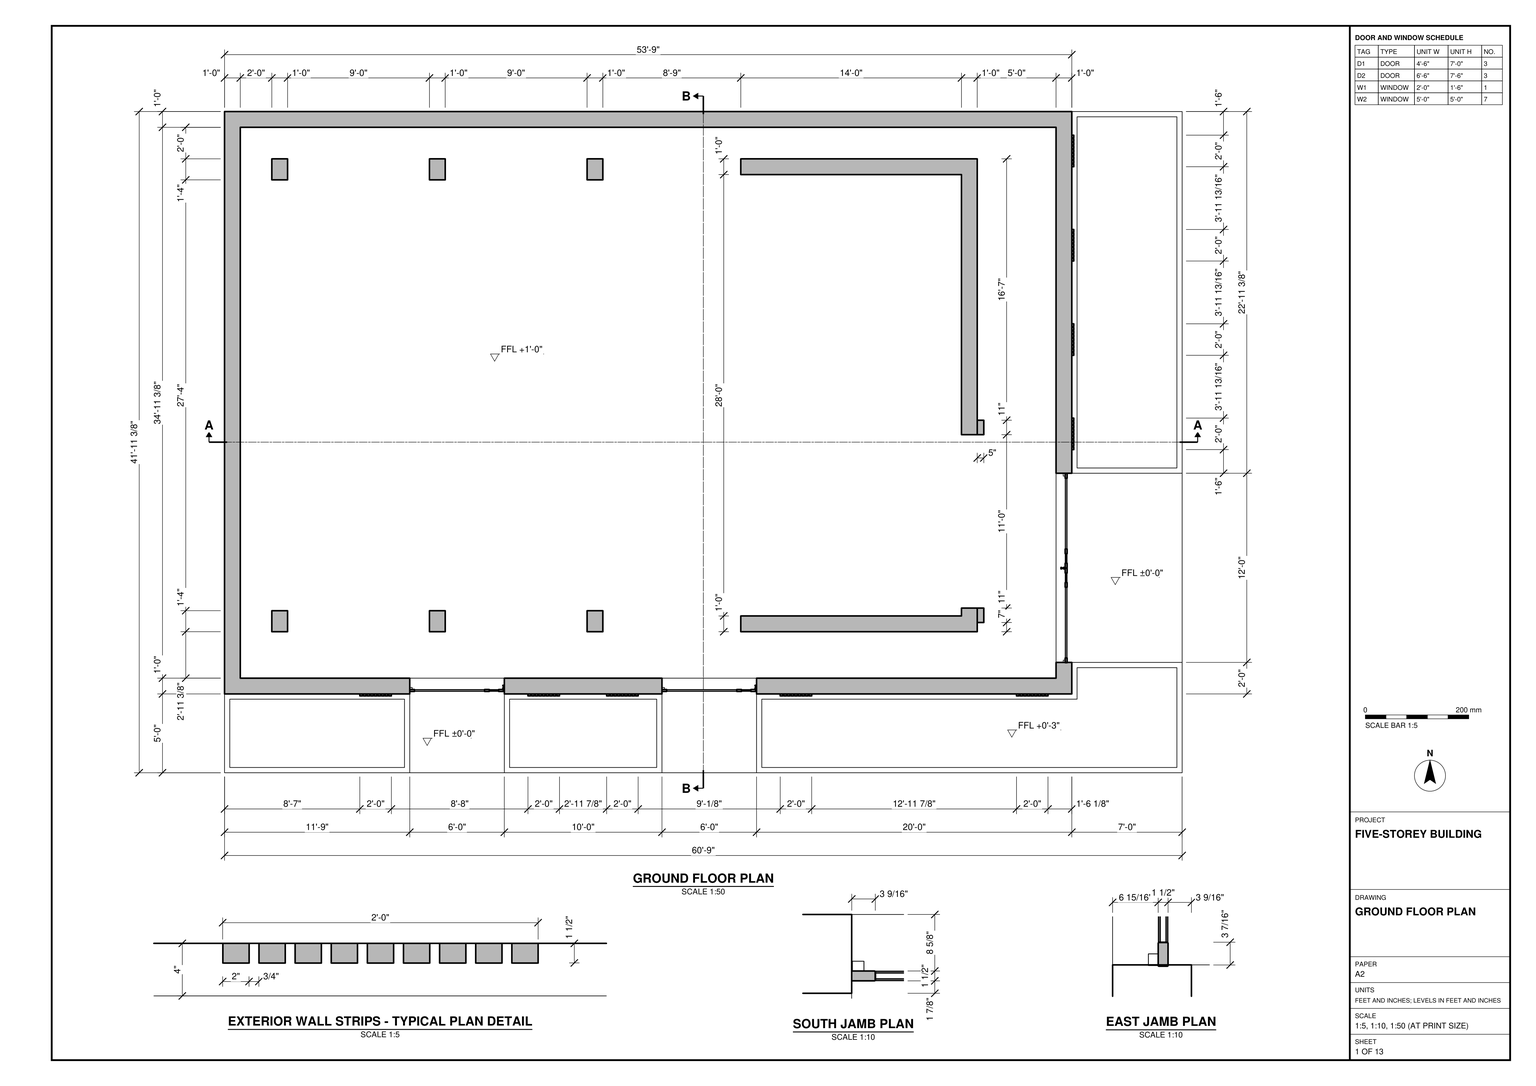
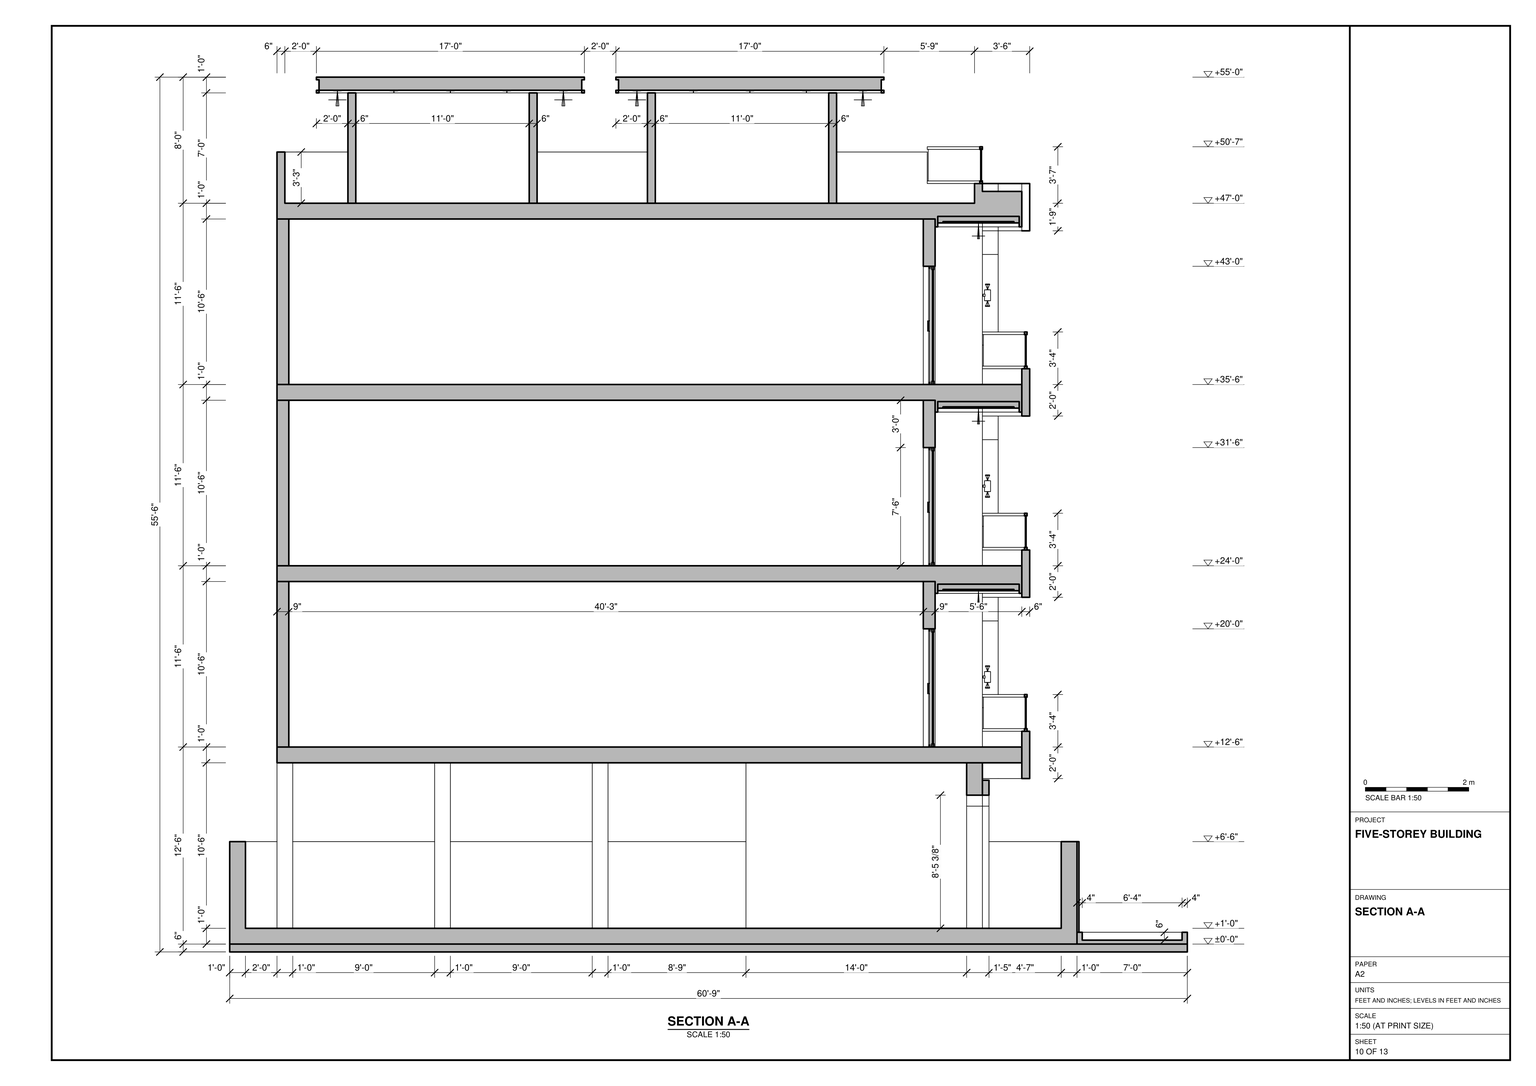
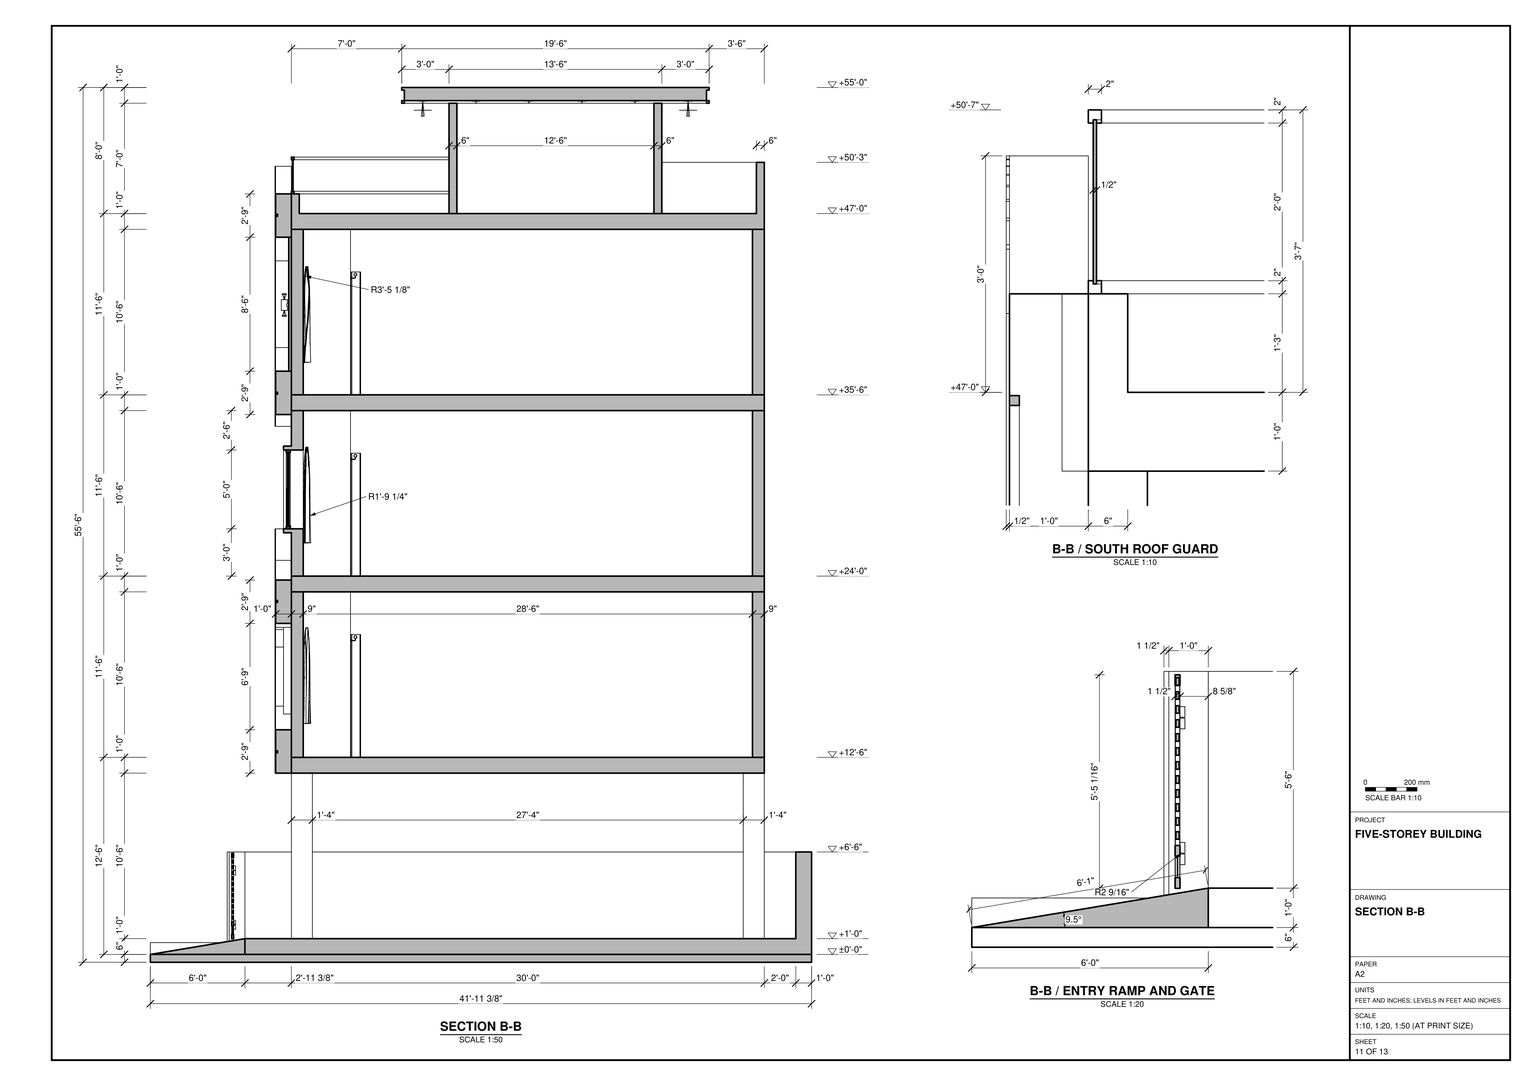
Build the building in SketchUp from task_files/diagram_01.pdf. Work in feet and inches. The complete model, including the base and rooftop canopies, measures 60'-9" east to west, 41'-11 3/8" north to south and 55'-6" from bottom to top. Use ±0'-0" as the ground datum and set the successive slab levels at +12'-6", +24'-0", +35'-6" and +47'-0". The last of these is the roof terrace, not the canopy top.

Start with the raised ground floor, low perimeter walls, entry ramps and gates. Keep the ground floor open around the two rows of freestanding columns, with the longer return wall and shorter wall in their plan positions to the east. Model the upper walls and slabs at the thicknesses drawn. Use the plans and opening schedule to place and size the doors and windows. Carry the east balconies beyond the enclosed floors and follow the sections for their slab edges and guards. On the roof, distinguish the solid parapets from the guarded edges and leave a gap between the two post-supported canopies. Include stairs, built-in joinery and main furniture only where shown on the sheets.

Keep walls, slabs, roof elements and each furniture or joinery piece in separate groups or components; use components for repeated parts. Decor and loose items may be any suitable library components. Save one SketchUp model as output_files/five_storey_building_with_balconies_and_roof_canopies.skp.

# SketchUp Ruby script. Lengths in inches.
U = 1.inch
M = Sketchup.active_model
def pt(a) = Geom::Point3d.new(a.map { |v| v * U })
def face(e, loops, mat)
  f = e.add_face(loops[0].map { |a| pt(a) })
  loops[1..].each { |l| e.add_face(l.map { |a| pt(a) }).erase! }
  f.material = f.back_material = mat if mat
  f
end
# faces: each face lists its corners as indices into pts; further lists are holes
def faces(e, pts, list, mat = nil) = list.each { |f| face(e, (f[0].is_a?(Array) ? f : [f]).map { |l| l.map { |i| pts[i] } }, mat) }
# xy, xz, yz: faces in a plane at the given z, y or x. An outline is a flat list of corners, or four numbers for a rectangle; further outlines are holes
def ring(l) = l.size == 4 ? [[l[0], l[1]], [l[2], l[1]], [l[2], l[3]], [l[0], l[3]]] : l.each_slice(2).to_a
def flat(e, list, mat, &to3) = list.each { |f| face(e, (f[0].is_a?(Array) ? f : [f]).map { |l| ring(l).map { |u, v| to3.(u, v) } }, mat) }
def xy(e, z, list, mat = nil) = flat(e, list, mat) { |x, y| [x, y, z] }
def xz(e, y, list, mat = nil) = flat(e, list, mat) { |x, z| [x, y, z] }
def yz(e, x, list, mat = nil) = flat(e, list, mat) { |y, z| [x, y, z] }
def lines(e, pts, list) = list.each { |a, b| e.add_line(pt(pts[a]), pt(pts[b])) }
# prism: a flat outline (further loops are holes) pulled along v
def prism(e, loops, v, mat = nil)
  f = face(e, loops, mat); d = Geom::Vector3d.new(v.map { |x| x * U })
  f.pushpull(f.normal.samedirection?(d) ? d.length : -d.length)
end
def box(e, o, s, mat = nil) = prism(e, [[o, [o[0] + s[0], o[1], o[2]], [o[0] + s[0], o[1] + s[1], o[2]], [o[0], o[1] + s[1], o[2]]]], [0, 0, s[2]], mat)
def at(x, y, z, deg = 0) = Geom::Transformation.translation(pt([x, y, z])) * Geom::Transformation.rotation(ORIGIN, Z_AXIS, deg.degrees)
def axes(o, x, y, z) = Geom::Transformation.new([*x, 0, *y, 0, *z, 0, *pt(o).to_a, 1])
def part(name) = M.definitions.add(name)
# library, detail: a bought-in or finely detailed component or shape, given as its bounding box
def library(name, o, s) = part(name).tap { |d| box(d.entities, o, s) }
def detail(e, o, s) = box(e.add_group.entities, o, s)
def put(e, d, t, mat = nil) = e.add_instance(d, t).tap { |i| i.material = mat if mat }
def group(e, t, mat = nil) = e.add_group.tap { |g| g.transformation = t; g.material = mat if mat }.entities
root = M.entities
M.materials.add("1111 AP 9939 Brown seed-N").color = [120, 84, 73]
M.materials.add("1432 AP 8245 TAR ROAD").color = [71, 72, 75]
M.materials.add("Generic").color = [172, 166, 153]
M.materials.add("W142X827B75_NILAYA IMAGINE 31756 ROLL B75").color = [192, 192, 189]
M.materials.add("[Brick Tumbled]").color = [135, 132, 132]
M.materials.add("[Granite Dark Gray]").color = [69, 68, 68]
M.materials.add("[Tile Travertine 2 inch]").color = [181, 178, 172]
M.materials.add("[Wood Cherry Original]").color = [152, 86, 42]
M.materials.add("[Wood Veneer 01]").color = [120, 70, 37]
c1 = library("BathRoom Window",[2.44,2.32,-1.4375],[28.18,2.86,36])
c2 = library("WALL LIGHT 69",[4.19,4.05,-8.78],[4.61,5.7,17.13])
c3 = library("2",[-24,-36,-9.91],[204,234,21.91])
c4 = library("Double slatted gate",[7.03,-128.55,-3.91],[5.33,99.02,60.06])
c5 = part("5")
box(c5.entities,[0,0,0],[12,16,126])
c6 = library("Group\#10",[-12,-12.5,-12],[99,12.5,186])
c7 = library("Double-hung window 69 in. x 58 in. triple row with mullions",[0,0,-3.59],[62,58,4.59])
c8 = library("Glass Door",[0,0,0],[72,3.54,96])
c9 = library("RIDEAUX \#16",[0,0,0],[103.86,7.74,93.57])
c10 = library("Curtain",[0,0,0],[121.12,7.86,100.24])
c11 = library("SLIDING+GLASS+DOOR",[0,-0.75,0],[72,5.75,80])
c12 = library("Group\#19",[0,0,0],[0.5,51,105])
c13 = library("Group\#46",[0,-2,0],[168,2,149.16])
c14 = library("Group\#20",[0,0,0],[0.5,51,102])
c15 = library("Group\#21",[0,0,0],[0.5,51,102])
c16 = library("Group\#58",[0,0,-17.09],[62,80,17.09])
c17 = library("Group\#32",[0,0,-17.09],[62,80,17.09])
c18 = library("Group\#56",[0,0,-17.09],[62,80,17.09])
c19 = library("Group\#9",[-9,-13,-20.09],[567,364,75.09])
c20 = library("Group\#3",[-12,-12.5,-24],[99,12.5,198])
c21 = library("Group\#17",[0,0,-12],[36,360,453])
c22 = library("Group\#13",[0,-12,0],[330,12,441])
c23 = library("Group\#18",[0,0,-453],[48,48,453])
c24 = library("Group\#45",[0,-2,0],[63,2,36])
c25 = library("Group\#43",[0,-2,0],[63,2,36])
c26 = library("Group\#47",[0,0,0],[34,92,28])
c27 = library("Group\#64",[0,-1.5,0],[24,1.5,78])
c28 = part("Group\#66")
prism(c28.entities,[[[0,-72,0],[0,0,12],[0,0,0]]],[72,0,0])
c29 = library("Group\#62",[0,0,0],[185,360,126])
c30 = library("Group\#1077",[59.37,-1.74,0],[60.38,4.74,59.75])
g1 = group(root,at(21,107.37,1.59))
g2 = group(g1,at(0,0,166.2))
box(g2,[-21,-107.37,-156],[729,503.37,6],"[Brick Tumbled]")
put(g2,c1,axes([456.92,-1.16,234.72],[0.85182,0,0],[0,0.5,0],[0,0,0.5]))
put(g2,c2,at(464.24,-13.25,184.26))
put(g2,c2,at(464.24,-13.25,328.62))
put(g2,c2,at(298.46,-11.75,344.61))
put(g2,c2,at(262.52,-9.75,203.46))
put(g2,c2,at(360.51,-9.75,62.87))
put(g2,c2,at(127.76,-9.75,62.87))
put(g2,c2,at(127.76,-9.75,193.87))
put(g2,c2,at(562.25,55.625,344.18,90))
put(g2,c2,at(562.25,55.625,198.87,90))
put(g2,c2,at(562.25,55.625,53.55,90))
put(g2,c2,at(562.25,268.01,344.18,90))
put(g2,c2,at(562.25,268.01,198.87,90))
put(g2,c2,at(562.25,268.01,53.55,90))
put(g2,c3,at(69,120,498))
put(g2,c3,at(297,120,498))
put(g2,c4,axes([628.05,163.36,-133.82],[-1,0,0],[0,1.45416,0],[0,0,1.06965]))
put(g2,c5,at(15,0,-138),"W142X827B75_NILAYA IMAGINE 31756 ROLL B75")
put(g2,c5,at(15,344,-138),"W142X827B75_NILAYA IMAGINE 31756 ROLL B75")
put(g2,c5,at(135,0,-138),"W142X827B75_NILAYA IMAGINE 31756 ROLL B75")
put(g2,c5,at(135,344,-138),"W142X827B75_NILAYA IMAGINE 31756 ROLL B75")
put(g2,c5,at(255,0,-138),"W142X827B75_NILAYA IMAGINE 31756 ROLL B75")
put(g2,c5,at(255,344,-138),"W142X827B75_NILAYA IMAGINE 31756 ROLL B75")
put(g2,c6,at(24,0,0),"[Wood Veneer 01]")
g3 = group(g2,at(15,-6,279))
xy(g3,-3,[[0,6,9,366],[93,6,537,15],[93,15,102,51],[528,15,528,135,492,135,492,147,501,147,501,144,537,144,537,15],[9,42,24,51],
  [78,42,93,51],[492,225,492,237,528,237,528,357,537,357,537,228,501,228,501,225],[9,357,537,366]])
xy(g3,30,[[138,0,204,6],[330,0,396,6]],"1111 AP 9939 Brown seed-N")
xy(g3,33,[[141,0,201,15],[333,0,393,15]],"1111 AP 9939 Brown seed-N")
xy(g3,81,[[24,42,78,51]])
xy(g3,87,[[492,147,501,225]])
xy(g3,93,[[333,0,393,15]])
xy(g3,93,[[141,0,201,15]],"1111 AP 9939 Brown seed-N")
xy(g3,96,[[138,0,204,6],[330,0,396,6]],"1111 AP 9939 Brown seed-N")
xy(g3,123,[[[0,6,9,6,9,42,93,42,93,6,537,6,537,144,501,144,501,228,537,228,537,366,0,366],[102,15,102,51,9,51,9,357,528,357,528,237,492,237,492,135,528,135,528,15]]])
xz(g3,0,[[[138,30,204,96],[141,33,201,93]],[[330,30,396,96],[333,33,393,93]]],"1111 AP 9939 Brown seed-N")
xz(g3,6,[[0,-3,9,123],[[93,-3,537,123],[330,30,396,96],[138,30,204,96]]])
xz(g3,15,[[[102,-3,528,123],[141,33,201,93],[333,33,393,93]]])
xz(g3,42,[[9,-3,24,-3,24,81,78,81,78,-3,93,-3,93,123,9,123]])
xz(g3,51,[[9,-3,9,123,102,123,102,-3,78,-3,78,81,24,81,24,-3]])
xz(g3,135,[[492,-3,528,123]])
xz(g3,144,[[501,-3,537,123]])
xz(g3,147,[[492,-3,501,87]])
xz(g3,225,[[492,-3,501,87]])
xz(g3,228,[[501,-3,537,123]])
xz(g3,237,[[492,-3,528,123]])
xz(g3,357,[[9,-3,528,123]])
xz(g3,366,[[0,-3,537,123]])
yz(g3,0,[[6,-3,366,123]])
yz(g3,9,[[6,-3,42,123],[51,-3,357,123]])
yz(g3,24,[[42,-3,51,81]])
yz(g3,78,[[42,-3,51,81]])
yz(g3,93,[[6,-3,42,123]])
yz(g3,102,[[15,-3,51,123]])
yz(g3,138,[[0,30,6,96]],"1111 AP 9939 Brown seed-N")
yz(g3,141,[[0,33,15,93]],"1111 AP 9939 Brown seed-N")
yz(g3,201,[[0,33,15,93]],"1111 AP 9939 Brown seed-N")
yz(g3,204,[[0,30,6,96]])
yz(g3,330,[[0,30,6,96]],"1111 AP 9939 Brown seed-N")
yz(g3,333,[[0,33,15,93]],"1111 AP 9939 Brown seed-N")
yz(g3,393,[[0,33,15,93]],"1111 AP 9939 Brown seed-N")
yz(g3,396,[[0,30,6,96]],"1111 AP 9939 Brown seed-N")
yz(g3,492,[[135,-3,135,123,237,123,237,-3,225,-3,225,87,147,87,147,-3]])
yz(g3,501,[[144,-3,147,-3,147,87,225,87,225,-3,228,-3,228,123,144,123]])
yz(g3,528,[[15,-3,135,123],[237,-3,357,123]])
yz(g3,537,[[59.76,9,93,9,93,114,59.76,114,59.53,113.99,59.29,113.99,59.06,113.98,58.82,113.96,58.59,113.94,58.35,113.92,58.12,113.9,57.88,113.875,57.65,113.85,57.42,113.8125,57.18,113.78,56.72,113.7,56.49,113.65,56.26,113.61,56.03,113.56,55.8,113.5,55.57,113.45,55.34,113.39,55.11,113.32,54.89,113.26,54.66,113.19,54.4375,113.12,54.21,113.04,53.99,112.97,53.77,112.89,53.55,112.8,53.33,112.72,52.89,112.54,52.68,112.44,52.46,112.35,52.25,112.25,52.04,112.14,51.83,112.04,51.41,111.82,51.2,111.7,51,111.59,50.6,111.35,50.39,111.22,50.2,111.1,50,110.97,49.8,110.83,49.61,110.7,49.42,110.5625,49.23,110.42,49.04,110.28,48.86,110.14,48.67,109.99,48.49,109.84,48.31,109.6875,48.13,109.53,47.96,109.375,47.78,109.22,47.61,109.06,47.44,108.89,47.27,108.73,47.11,108.56,46.94,108.39,46.78,108.22,46.625,108.04,46.47,107.87,46.3125,107.69,46.16,107.51,46.01,107.33,45.86,107.14,45.72,106.96,45.58,106.77,45.4375,106.58,45.3,106.39,45.17,106.2,45.03,106,44.9,105.8,44.78,105.61,44.65,105.4,44.41,105,44.3,104.8,44.18,104.59,43.96,104.17,43.86,103.96,43.75,103.75,43.65,103.54,43.56,103.32,43.46,103.11,43.28,102.67,43.2,102.45,43.11,102.23,43.03,102.01,42.96,101.79,42.88,101.5625,42.81,101.34,42.74,101.11,42.68,100.89,42.61,100.66,42.55,100.43,42.5,100.2,42.44,99.97,42.39,99.74,42.35,99.51,42.3,99.28,42.22,98.82,42.1875,98.58,42.15,98.35,42.125,98.12,42.1,97.88,42.08,97.65,42.06,97.41,42.04,97.18,42.02,96.94,42.01,96.71,42.01,96.47,42,96.24,42,26.76,42.01,26.53,42.01,26.29,42.02,26.06,42.04,25.82,42.06,25.59,42.08,25.35,42.1,25.12,42.125,24.88,42.15,24.65,42.1875,24.42,42.22,24.18,42.3,23.72,42.35,23.49,42.39,23.26,42.44,23.03,42.5,22.8,42.55,22.57,42.61,22.34,42.68,22.11,42.74,21.89,42.81,21.66,42.88,21.4375,42.96,21.21,43.03,20.99,43.11,20.77,43.2,20.55,43.28,20.33,43.46,19.89,43.56,19.68,43.65,19.46,43.75,19.25,43.86,19.04,43.96,18.83,44.18,18.41,44.3,18.2,44.41,18,44.65,17.6,44.78,17.39,44.9,17.2,45.03,17,45.17,16.8,45.3,16.61,45.4375,16.42,45.58,16.23,45.72,16.04,45.86,15.86,46.01,15.67,46.16,15.49,46.3125,15.31,46.47,15.13,46.625,14.96,46.78,14.78,46.94,14.61,47.11,14.44,47.27,14.27,47.44,14.11,47.61,13.94,47.78,13.78,47.96,13.625,48.13,13.47,48.31,13.3125,48.49,13.16,48.67,13.01,48.86,12.86,49.04,12.72,49.23,12.58,49.42,12.4375,49.61,12.3,49.8,12.17,50,12.03,50.2,11.9,50.39,11.78,50.6,11.65,51,11.41,51.2,11.3,51.41,11.18,51.83,10.96,52.04,10.86,52.25,10.75,52.46,10.65,52.68,10.56,52.89,10.46,53.33,10.28,53.55,10.2,53.77,10.11,53.99,10.03,54.21,9.96,54.4375,9.88,54.66,9.81,54.89,9.74,55.11,9.68,55.34,9.61,55.57,9.55,55.8,9.5,56.03,9.44,56.26,9.39,56.49,9.35,56.72,9.3,57.18,9.22,57.42,9.1875,57.65,9.15,57.88,9.125,58.12,9.1,58.35,9.08,58.59,9.06,58.82,9.04,59.06,9.02,59.29,9.01,59.53,9.01]])
yz(g3,537,[[[6,-3,144,123],[59.76,9,59.53,9.01,59.29,9.01,59.06,9.02,58.82,9.04,58.59,9.06,58.35,9.08,58.12,9.1,57.88,9.125,57.65,9.15,57.42,9.1875,57.18,9.22,56.72,9.3,56.49,9.35,56.26,9.39,56.03,9.44,55.8,9.5,55.57,9.55,55.34,9.61,55.11,9.68,54.89,9.74,54.66,9.81,54.4375,9.88,54.21,9.96,53.99,10.03,53.77,10.11,53.55,10.2,53.33,10.28,52.89,10.46,52.68,10.56,52.46,10.65,52.25,10.75,52.04,10.86,51.83,10.96,51.41,11.18,51.2,11.3,51,11.41,50.6,11.65,50.39,11.78,50.2,11.9,50,12.03,49.8,12.17,49.61,12.3,49.42,12.4375,49.23,12.58,49.04,12.72,48.86,12.86,48.67,13.01,48.49,13.16,48.31,13.3125,48.13,13.47,47.96,13.625,47.78,13.78,47.61,13.94,47.44,14.11,47.27,14.27,47.11,14.44,46.94,14.61,46.78,14.78,46.625,14.96,46.47,15.13,46.3125,15.31,46.16,15.49,46.01,15.67,45.86,15.86,45.72,16.04,45.58,16.23,45.4375,16.42,45.3,16.61,45.17,16.8,45.03,17,44.9,17.2,44.78,17.39,44.65,17.6,44.41,18,44.3,18.2,44.18,18.41,43.96,18.83,43.86,19.04,43.75,19.25,43.65,19.46,43.56,19.68,43.46,19.89,43.28,20.33,43.2,20.55,43.11,20.77,43.03,20.99,42.96,21.21,42.88,21.4375,42.81,21.66,42.74,21.89,42.68,22.11,42.61,22.34,42.55,22.57,42.5,22.8,42.44,23.03,42.39,23.26,42.35,23.49,42.3,23.72,42.22,24.18,42.1875,24.42,42.15,24.65,42.125,24.88,42.1,25.12,42.08,25.35,42.06,25.59,42.04,25.82,42.02,26.06,42.01,26.29,42.01,26.53,42,26.76,42,96.24,42.01,96.47,42.01,96.71,42.02,96.94,42.04,97.18,42.06,97.41,42.08,97.65,42.1,97.88,42.125,98.12,42.15,98.35,42.1875,98.58,42.22,98.82,42.3,99.28,42.35,99.51,42.39,99.74,42.44,99.97,42.5,100.2,42.55,100.43,42.61,100.66,42.68,100.89,42.74,101.11,42.81,101.34,42.88,101.5625,42.96,101.79,43.03,102.01,43.11,102.23,43.2,102.45,43.28,102.67,43.46,103.11,43.56,103.32,43.65,103.54,43.75,103.75,43.86,103.96,43.96,104.17,44.18,104.59,44.3,104.8,44.41,105,44.65,105.4,44.78,105.61,44.9,105.8,45.03,106,45.17,106.2,45.3,106.39,45.4375,106.58,45.58,106.77,45.72,106.96,45.86,107.14,46.01,107.33,46.16,107.51,46.3125,107.69,46.47,107.87,46.625,108.04,46.78,108.22,46.94,108.39,47.11,108.56,47.27,108.73,47.44,108.89,47.61,109.06,47.78,109.22,47.96,109.375,48.13,109.53,48.31,109.6875,48.49,109.84,48.67,109.99,48.86,110.14,49.04,110.28,49.23,110.42,49.42,110.5625,49.61,110.7,49.8,110.83,50,110.97,50.2,111.1,50.39,111.22,50.6,111.35,51,111.59,51.2,111.7,51.41,111.82,51.83,112.04,52.04,112.14,52.25,112.25,52.46,112.35,52.68,112.44,52.89,112.54,53.33,112.72,53.55,112.8,53.77,112.89,53.99,112.97,54.21,113.04,54.4375,113.12,54.66,113.19,54.89,113.26,55.11,113.32,55.34,113.39,55.57,113.45,55.8,113.5,56.03,113.56,56.26,113.61,56.49,113.65,56.72,113.7,57.18,113.78,57.42,113.8125,57.65,113.85,57.88,113.875,58.12,113.9,58.35,113.92,58.59,113.94,58.82,113.96,59.06,113.98,59.29,113.99,59.53,113.99,59.76,114,93,114,93,9]],[228,-3,366,123]],"Generic")
put(g3,c7,axes([201,4.5,33],[-0.96774,0,0],[0,0,1.03448],[0,0.696,0]),"[Granite Dark Gray]")
put(g3,c7,axes([393,4.5,33],[-0.96774,0,0],[0,0,1.03448],[0,0.696,0]),"[Granite Dark Gray]")
put(g3,c8,axes([24,42,-3],[0.75,0,0],[0,0.74,0],[0,0,0.875]))
put(g3,c9,axes([9,51,-3],[0.79912,0,0],[0,1,0],[0,0,1]))
put(g3,c10,axes([126.82,15,21.67],[0.73,0,0],[0,0.73,0],[0,0,0.73]))
put(g3,c10,axes([314.2,15,21.67],[0.73,0,0],[0,0.73,0],[0,0,0.73]))
put(g3,c11,axes([496,225,-3],[0,-1.08333,0],[1,0,0],[0,0,1.125]))
put(g3,c12,at(537,42,9),"[Wood Veneer 01]")
put(g3,c13,at(240,6,-32.16),"Generic")
g4 = group(g2,at(15,-6,141))
xy(g4,-3,[[0,6,0,366,528,366,528,357,9,357,9,51,24,51,24,42,9,42,9,6],[93,6,93,42,78,42,78,51,102,51,102,15,528,15,528,135,492,135,492,147,501,147,501,144,537,144,537,6],[492,225,492,237,528,237,528,366,537,366,537,228,501,228,501,225]])
xy(g4,30,[[138,0,204,6],[306,0,372,6]],"1111 AP 9939 Brown seed-N")
xy(g4,33,[[141,0,201,15],[309,0,369,15]],"1111 AP 9939 Brown seed-N")
xy(g4,81,[[24,42,78,51]])
xy(g4,87,[[492,147,501,225]])
xy(g4,93,[[444,6,468,15]])
xy(g4,93,[[141,0,201,15],[309,0,369,15]],"1111 AP 9939 Brown seed-N")
xy(g4,96,[[138,0,204,6],[306,0,372,6]],"1111 AP 9939 Brown seed-N")
xy(g4,111,[[444,6,468,15]])
xy(g4,123,[[[0,6,9,6,9,42,93,42,93,6,537,6,537,144,501,144,501,228,537,228,537,366,0,366],[102,15,102,51,9,51,9,357,528,357,528,237,492,237,492,135,528,135,528,15]]])
xz(g4,0,[[[138,30,204,96],[141,33,201,93]],[[306,30,372,96],[309,33,369,93]]],"1111 AP 9939 Brown seed-N")
xz(g4,6,[[0,-3,9,123],[[93,-3,537,123],[138,30,204,96],[306,30,372,96],[444,93,468,111]]])
xz(g4,15,[[[102,-3,528,123],[309,33,369,93],[141,33,201,93],[444,93,468,111]]])
xz(g4,42,[[9,-3,24,-3,24,81,78,81,78,-3,93,-3,93,123,9,123]])
xz(g4,51,[[9,-3,9,123,102,123,102,-3,78,-3,78,81,24,81,24,-3]])
xz(g4,135,[[492,-3,528,123]])
xz(g4,144,[[501,-3,537,123]])
xz(g4,147,[[492,-3,501,87]])
xz(g4,225,[[492,-3,501,87]])
xz(g4,228,[[501,-3,537,123]])
xz(g4,237,[[492,-3,528,123]])
xz(g4,357,[[9,-3,528,123]])
xz(g4,366,[[0,-3,537,123]])
yz(g4,0,[[6,-3,366,123]])
yz(g4,9,[[6,-3,42,123],[51,-3,357,123]])
yz(g4,24,[[42,-3,51,81]])
yz(g4,78,[[42,-3,51,81]])
yz(g4,93,[[6,-3,42,123]])
yz(g4,102,[[15,-3,51,123]])
yz(g4,138,[[0,30,6,96]],"1111 AP 9939 Brown seed-N")
yz(g4,141,[[0,33,15,93]],"1111 AP 9939 Brown seed-N")
yz(g4,201,[[0,33,15,93]],"1111 AP 9939 Brown seed-N")
yz(g4,204,[[0,30,6,96]],"1111 AP 9939 Brown seed-N")
yz(g4,306,[[0,30,6,96]],"1111 AP 9939 Brown seed-N")
yz(g4,309,[[0,33,15,93]],"1111 AP 9939 Brown seed-N")
yz(g4,369,[[0,33,15,93]],"1111 AP 9939 Brown seed-N")
yz(g4,372,[[0,30,6,96]])
yz(g4,444,[[6,93,15,111]])
yz(g4,468,[[6,93,15,111]])
yz(g4,492,[[135,-3,135,123,237,123,237,-3,225,-3,225,87,147,87,147,-3]])
yz(g4,501,[[144,-3,147,-3,147,87,225,87,225,-3,228,-3,228,123,144,123]])
yz(g4,528,[[15,-3,135,123],[237,-3,357,123]])
yz(g4,537,[[59.76,9,93,9,93,111,59.76,111,59.53,110.99,59.29,110.99,59.06,110.98,58.82,110.96,58.59,110.94,58.35,110.92,58.12,110.9,57.88,110.875,57.65,110.85,57.42,110.8125,57.18,110.78,56.72,110.7,56.49,110.65,56.26,110.61,56.03,110.56,55.8,110.5,55.57,110.45,55.34,110.39,55.11,110.32,54.89,110.26,54.66,110.19,54.4375,110.12,54.21,110.04,53.99,109.97,53.77,109.89,53.55,109.8,53.33,109.72,52.89,109.54,52.68,109.44,52.46,109.35,52.25,109.25,52.04,109.14,51.83,109.04,51.41,108.82,51.2,108.7,51,108.59,50.6,108.35,50.39,108.22,50.2,108.1,50,107.97,49.8,107.83,49.61,107.7,49.42,107.5625,49.23,107.42,49.04,107.28,48.86,107.14,48.67,106.99,48.49,106.84,48.31,106.6875,48.13,106.53,47.96,106.375,47.78,106.22,47.61,106.06,47.44,105.89,47.27,105.73,47.11,105.56,46.94,105.39,46.78,105.22,46.625,105.04,46.47,104.87,46.3125,104.69,46.16,104.51,46.01,104.33,45.86,104.14,45.72,103.96,45.58,103.77,45.4375,103.58,45.3,103.39,45.17,103.2,45.03,103,44.9,102.8,44.78,102.61,44.65,102.4,44.41,102,44.3,101.8,44.18,101.59,43.96,101.17,43.86,100.96,43.75,100.75,43.65,100.54,43.56,100.32,43.46,100.11,43.28,99.67,43.2,99.45,43.11,99.23,43.03,99.01,42.96,98.79,42.88,98.5625,42.81,98.34,42.74,98.11,42.68,97.89,42.61,97.66,42.55,97.43,42.5,97.2,42.44,96.97,42.39,96.74,42.35,96.51,42.3,96.28,42.22,95.82,42.1875,95.58,42.15,95.35,42.125,95.12,42.1,94.88,42.08,94.65,42.06,94.41,42.04,94.18,42.02,93.94,42.01,93.71,42.01,93.47,42,93.24,42,26.76,42.01,26.53,42.01,26.29,42.02,26.06,42.04,25.82,42.06,25.59,42.08,25.35,42.1,25.12,42.125,24.88,42.15,24.65,42.1875,24.42,42.22,24.18,42.3,23.72,42.35,23.49,42.39,23.26,42.44,23.03,42.5,22.8,42.55,22.57,42.61,22.34,42.68,22.11,42.74,21.89,42.81,21.66,42.88,21.4375,42.96,21.21,43.03,20.99,43.11,20.77,43.2,20.55,43.28,20.33,43.46,19.89,43.56,19.68,43.65,19.46,43.75,19.25,43.86,19.04,43.96,18.83,44.18,18.41,44.3,18.2,44.41,18,44.65,17.6,44.78,17.39,44.9,17.2,45.03,17,45.17,16.8,45.3,16.61,45.4375,16.42,45.58,16.23,45.72,16.04,45.86,15.86,46.01,15.67,46.16,15.49,46.3125,15.31,46.47,15.13,46.625,14.96,46.78,14.78,46.94,14.61,47.11,14.44,47.27,14.27,47.44,14.11,47.61,13.94,47.78,13.78,47.96,13.625,48.13,13.47,48.31,13.3125,48.49,13.16,48.67,13.01,48.86,12.86,49.04,12.72,49.23,12.58,49.42,12.4375,49.61,12.3,49.8,12.17,50,12.03,50.2,11.9,50.39,11.78,50.6,11.65,51,11.41,51.2,11.3,51.41,11.18,51.83,10.96,52.04,10.86,52.25,10.75,52.46,10.65,52.68,10.56,52.89,10.46,53.33,10.28,53.55,10.2,53.77,10.11,53.99,10.03,54.21,9.96,54.4375,9.88,54.66,9.81,54.89,9.74,55.11,9.68,55.34,9.61,55.57,9.55,55.8,9.5,56.03,9.44,56.26,9.39,56.49,9.35,56.72,9.3,57.18,9.22,57.42,9.1875,57.65,9.15,57.88,9.125,58.12,9.1,58.35,9.08,58.59,9.06,58.82,9.04,59.06,9.02,59.29,9.01,59.53,9.01]])
yz(g4,537,[[[6,-3,144,123],[59.76,9,59.53,9.01,59.29,9.01,59.06,9.02,58.82,9.04,58.59,9.06,58.35,9.08,58.12,9.1,57.88,9.125,57.65,9.15,57.42,9.1875,57.18,9.22,56.72,9.3,56.49,9.35,56.26,9.39,56.03,9.44,55.8,9.5,55.57,9.55,55.34,9.61,55.11,9.68,54.89,9.74,54.66,9.81,54.4375,9.88,54.21,9.96,53.99,10.03,53.77,10.11,53.55,10.2,53.33,10.28,52.89,10.46,52.68,10.56,52.46,10.65,52.25,10.75,52.04,10.86,51.83,10.96,51.41,11.18,51.2,11.3,51,11.41,50.6,11.65,50.39,11.78,50.2,11.9,50,12.03,49.8,12.17,49.61,12.3,49.42,12.4375,49.23,12.58,49.04,12.72,48.86,12.86,48.67,13.01,48.49,13.16,48.31,13.3125,48.13,13.47,47.96,13.625,47.78,13.78,47.61,13.94,47.44,14.11,47.27,14.27,47.11,14.44,46.94,14.61,46.78,14.78,46.625,14.96,46.47,15.13,46.3125,15.31,46.16,15.49,46.01,15.67,45.86,15.86,45.72,16.04,45.58,16.23,45.4375,16.42,45.3,16.61,45.17,16.8,45.03,17,44.9,17.2,44.78,17.39,44.65,17.6,44.41,18,44.3,18.2,44.18,18.41,43.96,18.83,43.86,19.04,43.75,19.25,43.65,19.46,43.56,19.68,43.46,19.89,43.28,20.33,43.2,20.55,43.11,20.77,43.03,20.99,42.96,21.21,42.88,21.4375,42.81,21.66,42.74,21.89,42.68,22.11,42.61,22.34,42.55,22.57,42.5,22.8,42.44,23.03,42.39,23.26,42.35,23.49,42.3,23.72,42.22,24.18,42.1875,24.42,42.15,24.65,42.125,24.88,42.1,25.12,42.08,25.35,42.06,25.59,42.04,25.82,42.02,26.06,42.01,26.29,42.01,26.53,42,26.76,42,93.24,42.01,93.47,42.01,93.71,42.02,93.94,42.04,94.18,42.06,94.41,42.08,94.65,42.1,94.88,42.125,95.12,42.15,95.35,42.1875,95.58,42.22,95.82,42.3,96.28,42.35,96.51,42.39,96.74,42.44,96.97,42.5,97.2,42.55,97.43,42.61,97.66,42.68,97.89,42.74,98.11,42.81,98.34,42.88,98.5625,42.96,98.79,43.03,99.01,43.11,99.23,43.2,99.45,43.28,99.67,43.46,100.11,43.56,100.32,43.65,100.54,43.75,100.75,43.86,100.96,43.96,101.17,44.18,101.59,44.3,101.8,44.41,102,44.65,102.4,44.78,102.61,44.9,102.8,45.03,103,45.17,103.2,45.3,103.39,45.4375,103.58,45.58,103.77,45.72,103.96,45.86,104.14,46.01,104.33,46.16,104.51,46.3125,104.69,46.47,104.87,46.625,105.04,46.78,105.22,46.94,105.39,47.11,105.56,47.27,105.73,47.44,105.89,47.61,106.06,47.78,106.22,47.96,106.375,48.13,106.53,48.31,106.6875,48.49,106.84,48.67,106.99,48.86,107.14,49.04,107.28,49.23,107.42,49.42,107.5625,49.61,107.7,49.8,107.83,50,107.97,50.2,108.1,50.39,108.22,50.6,108.35,51,108.59,51.2,108.7,51.41,108.82,51.83,109.04,52.04,109.14,52.25,109.25,52.46,109.35,52.68,109.44,52.89,109.54,53.33,109.72,53.55,109.8,53.77,109.89,53.99,109.97,54.21,110.04,54.4375,110.12,54.66,110.19,54.89,110.26,55.11,110.32,55.34,110.39,55.57,110.45,55.8,110.5,56.03,110.56,56.26,110.61,56.49,110.65,56.72,110.7,57.18,110.78,57.42,110.8125,57.65,110.85,57.88,110.875,58.12,110.9,58.35,110.92,58.59,110.94,58.82,110.96,59.06,110.98,59.29,110.99,59.53,110.99,59.76,111,93,111,93,9]],[228,-3,366,123]],"Generic")
put(g4,c7,axes([201,4.5,33],[-0.96774,0,0],[0,0,1.03448],[0,0.696,0]),"[Granite Dark Gray]")
put(g4,c7,axes([369,4.5,33],[-0.96774,0,0],[0,0,1.03448],[0,0.696,0]),"[Granite Dark Gray]")
put(g4,c8,axes([24,42,-3],[0.75,0,0],[0,0.74,0],[0,0,0.875]))
put(g4,c9,axes([9,51,-3],[0.79912,0,0],[0,1,0],[0,0,1]))
put(g4,c10,axes([127.26,15,22.18],[0.73,0,0],[0,0.73,0],[0,0,0.73]))
put(g4,c10,axes([292.51,15,22.18],[0.73,0,0],[0,0.73,0],[0,0,0.73]))
put(g4,c11,axes([496,225,-3],[0,-1.08333,0],[1,0,0],[0,0,1.125]))
put(g4,c14,at(537,42,9),"[Wood Veneer 01]")
g5 = group(g2,at(15,-6,0))
xy(g5,0,[[0,6,0,366,537,366,537,228,501,228,501,225,492,225,492,234,528,234,528,357,9,357,9,51,24,51,24,42,9,42,9,6],[93,6,93,42,78,42,78,51,102,51,102,15,528,15,528,135,492,135,492,147,501,147,501,144,537,144,537,6]])
xy(g5,33,[[138,0,204,6],[246,0,312,6],[390,0,456,6]],"1111 AP 9939 Brown seed-N")
xy(g5,36,[[141,0,201,15],[249,0,309,15],[393,0,453,15]],"1111 AP 9939 Brown seed-N")
xy(g5,84,[[24,42,78,51]])
xy(g5,90,[[492,147,501,225]])
xy(g5,96,[[141,0,201,15],[249,0,309,15],[393,0,453,15]],"1111 AP 9939 Brown seed-N")
xy(g5,99,[[138,0,204,6],[246,0,312,6],[390,0,456,6]],"1111 AP 9939 Brown seed-N")
xy(g5,126,[[[0,6,9,6,9,42,93,42,93,6,537,6,537,144,501,144,501,228,537,228,537,366,0,366],[102,15,102,51,9,51,9,357,528,357,528,234,492,234,492,135,528,135,528,15]]])
xz(g5,0,[[[138,33,204,99],[141,36,201,96]],[[246,33,312,99],[249,36,309,96]],[[390,33,456,99],[393,36,453,96]]],"1111 AP 9939 Brown seed-N")
xz(g5,6,[[0,0,9,126],[[93,0,537,126],[138,33,204,99],[246,33,312,99],[390,33,456,99]]])
xz(g5,15,[[[102,0,528,126],[141,36,201,96],[249,36,309,96],[393,36,453,96]]])
xz(g5,42,[[9,0,24,0,24,84,78,84,78,0,93,0,93,126,9,126]])
xz(g5,51,[[9,0,9,126,102,126,102,0,78,0,78,84,24,84,24,0]])
xz(g5,135,[[492,0,528,126]])
xz(g5,144,[[501,0,537,126]])
xz(g5,147,[[492,0,501,90]])
xz(g5,225,[[492,0,501,90]])
xz(g5,228,[[501,0,537,126]])
xz(g5,234,[[492,0,528,126]])
xz(g5,357,[[9,0,528,126]])
xz(g5,366,[[0,0,537,126]])
yz(g5,0,[[6,0,366,126]])
yz(g5,9,[[6,0,42,126],[51,0,357,126]])
yz(g5,24,[[42,0,51,84]])
yz(g5,78,[[42,0,51,84]])
yz(g5,93,[[6,0,42,126]])
yz(g5,102,[[15,0,51,126]])
yz(g5,138,[[0,33,6,99]],"[Wood Veneer 01]")
yz(g5,141,[[0,36,15,96]],"1111 AP 9939 Brown seed-N")
yz(g5,201,[[0,36,15,96]],"1111 AP 9939 Brown seed-N")
yz(g5,204,[[0,33,6,99]],"1111 AP 9939 Brown seed-N")
yz(g5,246,[[0,33,6,99]],"1111 AP 9939 Brown seed-N")
yz(g5,249,[[0,36,15,96]],"1111 AP 9939 Brown seed-N")
yz(g5,309,[[0,36,15,96]],"1111 AP 9939 Brown seed-N")
yz(g5,312,[[0,33,6,99]],"1111 AP 9939 Brown seed-N")
yz(g5,390,[[0,33,6,99]],"1111 AP 9939 Brown seed-N")
yz(g5,393,[[0,36,15,96]],"1111 AP 9939 Brown seed-N")
yz(g5,453,[[0,36,15,96]],"1111 AP 9939 Brown seed-N")
yz(g5,456,[[0,33,6,99]],"1111 AP 9939 Brown seed-N")
yz(g5,492,[[135,0,135,126,234,126,234,0,225,0,225,90,147,90,147,0]])
yz(g5,501,[[144,0,147,0,147,90,225,90,225,0,228,0,228,126,144,126]])
yz(g5,528,[[15,0,135,126],[234,0,357,126]])
yz(g5,537,[[[6,0,144,126],[59.76,12,59.53,12.01,59.29,12.01,59.06,12.02,58.82,12.04,58.59,12.06,58.35,12.08,58.12,12.1,57.88,12.125,57.65,12.15,57.42,12.1875,57.18,12.22,56.72,12.3,56.49,12.35,56.26,12.39,56.03,12.44,55.8,12.5,55.57,12.55,55.34,12.61,55.11,12.68,54.89,12.74,54.66,12.81,54.4375,12.88,54.21,12.96,53.99,13.03,53.77,13.11,53.55,13.2,53.33,13.28,52.89,13.46,52.68,13.56,52.46,13.65,52.25,13.75,52.04,13.86,51.83,13.96,51.41,14.18,51.2,14.3,51,14.41,50.6,14.65,50.39,14.78,50.2,14.9,50,15.03,49.8,15.17,49.61,15.3,49.42,15.4375,49.23,15.58,49.04,15.72,48.86,15.86,48.67,16.01,48.49,16.16,48.31,16.3125,48.13,16.47,47.96,16.625,47.78,16.78,47.61,16.94,47.44,17.11,47.27,17.27,47.11,17.44,46.94,17.61,46.78,17.78,46.625,17.96,46.47,18.13,46.3125,18.31,46.16,18.49,46.01,18.67,45.86,18.86,45.72,19.04,45.58,19.23,45.4375,19.42,45.3,19.61,45.17,19.8,45.03,20,44.9,20.2,44.78,20.39,44.65,20.6,44.41,21,44.3,21.2,44.18,21.41,43.96,21.83,43.86,22.04,43.75,22.25,43.65,22.46,43.56,22.68,43.46,22.89,43.28,23.33,43.2,23.55,43.11,23.77,43.03,23.99,42.96,24.21,42.88,24.4375,42.81,24.66,42.74,24.89,42.68,25.11,42.61,25.34,42.55,25.57,42.5,25.8,42.44,26.03,42.39,26.26,42.35,26.49,42.3,26.72,42.22,27.18,42.1875,27.42,42.15,27.65,42.125,27.88,42.1,28.12,42.08,28.35,42.06,28.59,42.04,28.82,42.02,29.06,42.01,29.29,42.01,29.53,42,29.76,42,96.24,42.01,96.47,42.01,96.71,42.02,96.94,42.04,97.18,42.06,97.41,42.08,97.65,42.1,97.88,42.125,98.12,42.15,98.35,42.1875,98.58,42.22,98.82,42.3,99.28,42.35,99.51,42.39,99.74,42.44,99.97,42.5,100.2,42.55,100.43,42.61,100.66,42.68,100.89,42.74,101.11,42.81,101.34,42.88,101.5625,42.96,101.79,43.03,102.01,43.11,102.23,43.2,102.45,43.28,102.67,43.46,103.11,43.56,103.32,43.65,103.54,43.75,103.75,43.86,103.96,43.96,104.17,44.18,104.59,44.3,104.8,44.41,105,44.65,105.4,44.78,105.61,44.9,105.8,45.03,106,45.17,106.2,45.3,106.39,45.4375,106.58,45.58,106.77,45.72,106.96,45.86,107.14,46.01,107.33,46.16,107.51,46.3125,107.69,46.47,107.87,46.625,108.04,46.78,108.22,46.94,108.39,47.11,108.56,47.27,108.73,47.44,108.89,47.61,109.06,47.78,109.22,47.96,109.375,48.13,109.53,48.31,109.6875,48.49,109.84,48.67,109.99,48.86,110.14,49.04,110.28,49.23,110.42,49.42,110.5625,49.61,110.7,49.8,110.83,50,110.97,50.2,111.1,50.39,111.22,50.6,111.35,51,111.59,51.2,111.7,51.41,111.82,51.83,112.04,52.04,112.14,52.25,112.25,52.46,112.35,52.68,112.44,52.89,112.54,53.33,112.72,53.55,112.8,53.77,112.89,53.99,112.97,54.21,113.04,54.4375,113.12,54.66,113.19,54.89,113.26,55.11,113.32,55.34,113.39,55.57,113.45,55.8,113.5,56.03,113.56,56.26,113.61,56.49,113.65,56.72,113.7,57.18,113.78,57.42,113.8125,57.65,113.85,57.88,113.875,58.12,113.9,58.35,113.92,58.59,113.94,58.82,113.96,59.06,113.98,59.29,113.99,59.53,113.99,59.76,114,93,114,93,12]],[228,0,366,126]],"Generic")
yz(g5,537,[[59.76,12,93,12,93,114,59.76,114,59.53,113.99,59.29,113.99,59.06,113.98,58.82,113.96,58.59,113.94,58.35,113.92,58.12,113.9,57.88,113.875,57.65,113.85,57.42,113.8125,57.18,113.78,56.72,113.7,56.49,113.65,56.26,113.61,56.03,113.56,55.8,113.5,55.57,113.45,55.34,113.39,55.11,113.32,54.89,113.26,54.66,113.19,54.4375,113.12,54.21,113.04,53.99,112.97,53.77,112.89,53.55,112.8,53.33,112.72,52.89,112.54,52.68,112.44,52.46,112.35,52.25,112.25,52.04,112.14,51.83,112.04,51.41,111.82,51.2,111.7,51,111.59,50.6,111.35,50.39,111.22,50.2,111.1,50,110.97,49.8,110.83,49.61,110.7,49.42,110.5625,49.23,110.42,49.04,110.28,48.86,110.14,48.67,109.99,48.49,109.84,48.31,109.6875,48.13,109.53,47.96,109.375,47.78,109.22,47.61,109.06,47.44,108.89,47.27,108.73,47.11,108.56,46.94,108.39,46.78,108.22,46.625,108.04,46.47,107.87,46.3125,107.69,46.16,107.51,46.01,107.33,45.86,107.14,45.72,106.96,45.58,106.77,45.4375,106.58,45.3,106.39,45.17,106.2,45.03,106,44.9,105.8,44.78,105.61,44.65,105.4,44.41,105,44.3,104.8,44.18,104.59,43.96,104.17,43.86,103.96,43.75,103.75,43.65,103.54,43.56,103.32,43.46,103.11,43.28,102.67,43.2,102.45,43.11,102.23,43.03,102.01,42.96,101.79,42.88,101.5625,42.81,101.34,42.74,101.11,42.68,100.89,42.61,100.66,42.55,100.43,42.5,100.2,42.44,99.97,42.39,99.74,42.35,99.51,42.3,99.28,42.22,98.82,42.1875,98.58,42.15,98.35,42.125,98.12,42.1,97.88,42.08,97.65,42.06,97.41,42.04,97.18,42.02,96.94,42.01,96.71,42.01,96.47,42,96.24,42,29.76,42.01,29.53,42.01,29.29,42.02,29.06,42.04,28.82,42.06,28.59,42.08,28.35,42.1,28.12,42.125,27.88,42.15,27.65,42.1875,27.42,42.22,27.18,42.3,26.72,42.35,26.49,42.39,26.26,42.44,26.03,42.5,25.8,42.55,25.57,42.61,25.34,42.68,25.11,42.74,24.89,42.81,24.66,42.88,24.4375,42.96,24.21,43.03,23.99,43.11,23.77,43.2,23.55,43.28,23.33,43.46,22.89,43.56,22.68,43.65,22.46,43.75,22.25,43.86,22.04,43.96,21.83,44.18,21.41,44.3,21.2,44.41,21,44.65,20.6,44.78,20.39,44.9,20.2,45.03,20,45.17,19.8,45.3,19.61,45.4375,19.42,45.58,19.23,45.72,19.04,45.86,18.86,46.01,18.67,46.16,18.49,46.3125,18.31,46.47,18.13,46.625,17.96,46.78,17.78,46.94,17.61,47.11,17.44,47.27,17.27,47.44,17.11,47.61,16.94,47.78,16.78,47.96,16.625,48.13,16.47,48.31,16.3125,48.49,16.16,48.67,16.01,48.86,15.86,49.04,15.72,49.23,15.58,49.42,15.4375,49.61,15.3,49.8,15.17,50,15.03,50.2,14.9,50.39,14.78,50.6,14.65,51,14.41,51.2,14.3,51.41,14.18,51.83,13.96,52.04,13.86,52.25,13.75,52.46,13.65,52.68,13.56,52.89,13.46,53.33,13.28,53.55,13.2,53.77,13.11,53.99,13.03,54.21,12.96,54.4375,12.88,54.66,12.81,54.89,12.74,55.11,12.68,55.34,12.61,55.57,12.55,55.8,12.5,56.03,12.44,56.26,12.39,56.49,12.35,56.72,12.3,57.18,12.22,57.42,12.1875,57.65,12.15,57.88,12.125,58.12,12.1,58.35,12.08,58.59,12.06,58.82,12.04,59.06,12.02,59.29,12.01,59.53,12.01]],"[Wood Veneer 01]")
put(g5,c7,axes([201,4.5,36],[-0.96774,0,0],[0,0,1.03448],[0,0.696,0]),"[Granite Dark Gray]")
put(g5,c7,axes([309,4.5,36],[-0.96774,0,0],[0,0,1.03448],[0,0.696,0]),"[Granite Dark Gray]")
put(g5,c7,axes([453,4.5,36],[-0.96774,0,0],[0,0,1.03448],[0,0.696,0]),"[Granite Dark Gray]")
put(g5,c8,axes([24,42,0],[0.75,0,0],[0,0.74,0],[0,0,0.875]))
put(g5,c9,axes([9,51,0],[0.79912,0,0],[0,1,0],[0,0,1]))
put(g5,c10,axes([126.25,15,25.6875],[0.73,0,0],[0,0.73,0],[0,0,0.73]))
put(g5,c10,axes([234.25,15,25.6875],[0.73,0,0],[0,0.73,0],[0,0,0.73]))
put(g5,c10,axes([377,15,25.6875],[0.73,0,0],[0,0.73,0],[0,0,0.73]))
put(g5,c11,axes([496,225,0],[0,-1.08333,0],[1,0,0],[0,0,1.125]))
put(g5,c15,at(537,42,12),"[Wood Veneer 01]")
g6 = group(g2,at(24,9,126))
xy(g6,-9,[[[0,-9,84,27],[2,-7,82,25]],[[492,129,558,213],[494,131,556,211]]])
xy(g6,-3,[[2,-7,82,25]])
xy(g6,-2,[[494,131,556,211]])
xy(g6,0,[[-9,-9,-9,351,528,351,528,213,492,213,492,129,528,129,528,-9,84,-9,84,27,0,27,0,-9]])
xy(g6,12,[[-9,-9,528,-9,528,129,558,129,558,213,528,213,528,351,-9,351]])
xz(g6,-9,[[0,-9,84,12],[-9,0,0,12],[84,0,528,12]])
xz(g6,-7,[[2,-9,82,-3]])
xz(g6,25,[[2,-9,82,-3]])
xz(g6,27,[[0,-9,84,0]])
xz(g6,129,[[492,-9,528,0],[528,-9,558,12]])
xz(g6,131,[[494,-9,556,-2]])
xz(g6,211,[[494,-9,556,-2]])
xz(g6,213,[[492,-9,528,0],[528,-9,558,12]])
xz(g6,351,[[-9,0,528,12]])
yz(g6,-9,[[-9,0,351,12]])
yz(g6,0,[[-9,-9,27,0]])
yz(g6,2,[[-7,-9,25,-3]])
yz(g6,82,[[-7,-9,25,-3]])
yz(g6,84,[[-9,-9,27,0]])
yz(g6,492,[[129,-9,213,0]])
yz(g6,494,[[131,-9,211,-2]])
yz(g6,528,[[-9,0,129,12],[[213,0,351,12],[216.39,3.39,347.61,8.61]],[216.39,3.39,347.61,8.61]])
yz(g6,556,[[131,-9,211,-2]])
yz(g6,558,[[129,-9,213,12]])
put(g6,c16,at(494,131,-2))
put(g6,c17,axes([2,25,-3],[0,-0.54839,0],[1,0,0],[0,0,1]))
g7 = group(g2,at(24,9,264))
xy(g7,-9,[[[0,-9,84,27],[2,-7,82,25]],[[492,129,558,213],[494,131,556,211]]])
xy(g7,-3,[[2,-7,82,25]])
xy(g7,-1,[[494,131,556,211]])
xy(g7,0,[[-9,-9,-9,351,528,351,528,213,492,213,492,129,528,129,528,-9,84,-9,84,27,0,27,0,-9]])
xy(g7,12,[[-9,-9,528,-9,528,129,558,129,558,213,528,213,528,351,-9,351]])
xz(g7,-9,[[0,-9,84,-9,84,0,528,0,528,12,-9,12,-9,0,0,0]])
xz(g7,-7,[[2,-9,82,-3]])
xz(g7,25,[[2,-9,82,-3]])
xz(g7,27,[[0,-9,84,0]])
xz(g7,129,[[492,-9,528,0],[528,-9,558,12]])
xz(g7,131,[[494,-9,528,-1],[528,-9,556,-1]])
xz(g7,211,[[494,-9,528,-1],[528,-9,556,-1]])
xz(g7,213,[[492,-9,528,0],[528,-9,558,12]])
xz(g7,351,[[-9,0,528,12]])
yz(g7,-9,[[-9,0,351,12]])
yz(g7,0,[[-9,-9,27,0]])
yz(g7,2,[[-7,-9,25,-3]])
yz(g7,82,[[-7,-9,25,-3]])
yz(g7,84,[[-9,-9,27,0]])
yz(g7,492,[[129,-9,213,0]])
yz(g7,494,[[131,-9,211,-1]])
yz(g7,528,[[-9,0,129,12],[213,0,351,12]])
yz(g7,556,[[131,-9,211,-1]])
yz(g7,558,[[129,-9,213,12]])
put(g7,c18,at(494,131,-1))
put(g7,c17,axes([2,25,-3],[0,-0.54839,0],[1,0,0],[0,0,1]))
put(g2,c19,at(24,9,402))
put(g2,c20,at(24,0,276),"[Wood Veneer 01]")
g8 = group(g2,at(24,9,-12))
prism(g8,[[[-9,-9,0],[-9,351,0],[528,351,0],[528,213,0],[558,213,0],[558,129,0],[528,129,0],[528,-9,0],[84,-9,0],[0,-9,0]]],[0,0,12])
put(g2,c21,at(552,0,-12),"1432 AP 8245 TAR ROAD")
put(g2,c22,at(222,0,-12),"1432 AP 8245 TAR ROAD")
put(g2,c23,at(516,-12,429),"1432 AP 8245 TAR ROAD")
put(g2,c24,at(30,-6.5,276),"[Wood Cherry Original]")
put(g2,c25,at(30,-7,0),"[Wood Cherry Original]")
put(g2,c26,at(552,134,288),"[Wood Cherry Original]")
put(g2,c26,at(552,134,150),"[Wood Cherry Original]")
put(g2,c26,at(552,134,12),"[Wood Cherry Original]")
put(g2,c25,at(30,-7,138),"[Wood Cherry Original]")
g9 = group(g2,at(69,120,414),"Generic")
prism(g9,[[[0,0,0],[0,162,0],[144,162,0],[144,0,0]],[[6,156,0],[6,6,0],[138,6,0],[138,156,0]]],[0,0,84])
prism(g9,[[[228,162,0],[372,162,0],[372,0,0],[228,0,0]],[[234,156,0],[234,6,0],[366,6,0],[366,156,0]]],[0,0,84])
g10 = group(g2,at(15,-11.37,-138))
xy(g10,-12,[[-36,-36,-36,407.37,609,407.37,609,132,597,132,597,-12,609,-12,609,-36,369,-36,369,-24,297,-24,297,-36,177,-36,177,-24,105,-24,105,-36]])
xy(g10,0,[[-24,-24,597,395.37]],"[Tile Travertine 2 inch]")
xy(g10,66,[[-36,-36,105,-36,105,-24,-24,-24,-24,395.37,597,395.37,597,132,609,132,609,407.37,-36,407.37],[177,-36,297,-24],[369,-36,609,-36,609,-12,597,-12,597,-24,369,-24]])
xz(g10,-36,[[-36,-12,105,66],[177,-12,297,66],[369,-12,609,66]])
xz(g10,-24,[[105,-12,177,0],[297,-12,369,0],[-24,0,105,66],[177,0,297,66],[369,0,597,66]])
xz(g10,-12,[[597,-12,609,66]])
xz(g10,132,[[597,-12,609,66]])
xz(g10,395.37,[[-24,0,597,66]])
xz(g10,407.37,[[-36,-12,609,66]])
yz(g10,-36,[[-36,-12,407.37,66]])
yz(g10,-24,[[-24,0,395.37,66]])
yz(g10,105,[[-36,-12,-24,66]])
yz(g10,177,[[-36,-12,-24,66]])
yz(g10,297,[[-36,-12,-24,66]])
yz(g10,369,[[-36,-12,-24,66]])
yz(g10,597,[[-12,-12,132,0],[-24,0,-12,66],[132,0,395.37,66]])
yz(g10,609,[[-36,-12,-12,66],[132,-12,407.37,66]])
put(g10,c27,axes([387,-36,-3],[1,0,0],[0,1,0],[0,0,0.88462]),"[Wood Veneer 01]")
put(g10,c27,axes([566.875,-36,-3],[1,0,0],[0,1,0],[0,0,0.88462]),"[Wood Veneer 01]")
put(g10,c27,axes([254.875,-36,-3],[1,0,0],[0,1,0],[0,0,0.88462]),"[Wood Veneer 01]")
put(g10,c27,axes([195,-36,-3],[1,0,0],[0,1,0],[0,0,0.88462]),"[Wood Veneer 01]")
put(g10,c27,axes([67,-36,-3],[1,0,0],[0,1,0],[0,0,0.88462]),"[Wood Veneer 01]")
put(g10,c27,axes([609,150,-3],[0,1,0],[-1,0,0],[0,0,0.88462]),"[Wood Veneer 01]")
put(g10,c27,axes([609,365.37,-3],[0,1,0],[-1,0,0],[0,0,0.88462]),"[Wood Veneer 01]")
put(g10,c27,axes([609,221.79,-3],[0,1,0],[-1,0,0],[0,0,0.88462]),"[Wood Veneer 01]")
put(g10,c27,axes([609,293.58,-3],[0,1,0],[-1,0,0],[0,0,0.88462]),"[Wood Veneer 01]")
g11 = group(g10,at(597,-12,-12),"[Tile Travertine 2 inch]")
prism(g11,[[[0,144,0],[0,144,12],[96,144,0]]],[0,-144,0])
put(g10,c28,at(297,-24,-12),"[Tile Travertine 2 inch]")
put(g10,c28,at(105,-24,-12),"[Tile Travertine 2 inch]")
put(g2,c29,at(372,0,-138))
g12 = group(g2,at(-21,-107.37,-150),"[Brick Tumbled]")
xy(g12,0,[[0,0,141,60],[213,0,333,60],[405,0,405,60,645,60,645,84,729,84,729,0],[645,228,729,503.37]])
xy(g12,3,[[4,4,137,56],[217,4,329,56],[409,4,725,4,725,80,649,80,649,56,409,56],[649,232,725,499.37]])
xy(g12,9,[[[0,0,141,60],[4,4,137,56]],[[213,0,333,60],[217,4,329,56]],[[405,0,729,0,729,84,645,84,645,60,405,60],[409,4,409,56,649,56,649,80,725,80,725,4]],[[645,228,729,503.37],[649,232,725,499.37]]])
xz(g12,0,[[0,0,141,9],[213,0,333,9],[405,0,729,9]])
xz(g12,4,[[4,3,137,9],[217,3,329,9],[409,3,725,9]])
xz(g12,56,[[4,3,137,9],[217,3,329,9],[409,3,649,9]])
xz(g12,60,[[0,0,141,9],[213,0,333,9],[405,0,645,9]])
xz(g12,80,[[649,3,725,9]])
xz(g12,84,[[645,0,729,9]])
xz(g12,228,[[645,0,729,9]])
xz(g12,232,[[649,3,725,9]])
xz(g12,499.37,[[649,3,725,9]])
xz(g12,503.37,[[645,0,729,9]])
yz(g12,0,[[0,0,60,9]])
yz(g12,4,[[4,3,56,9]])
yz(g12,137,[[4,3,56,9]])
yz(g12,141,[[0,0,60,9]])
yz(g12,213,[[0,0,60,9]])
yz(g12,217,[[4,3,56,9]])
yz(g12,329,[[4,3,56,9]])
yz(g12,333,[[0,0,60,9]])
yz(g12,405,[[0,0,60,9]])
yz(g12,409,[[4,3,56,9]])
yz(g12,645,[[60,0,84,9],[228,0,503.37,9]])
yz(g12,649,[[56,3,80,9],[232,3,499.37,9]])
yz(g12,725,[[4,3,80,9],[232,3,499.37,9]])
yz(g12,729,[[0,0,84,9],[228,0,503.37,9]])
put(g2,c30,axes([454.8,-42.48,-138.07],[-1.19247,0,0],[0,-1,0],[0,0,1.08855]))
put(g2,c30,axes([262.8,-42.48,-138.07],[-1.19247,0,0],[0,-1,0],[0,0,1.08855]))
